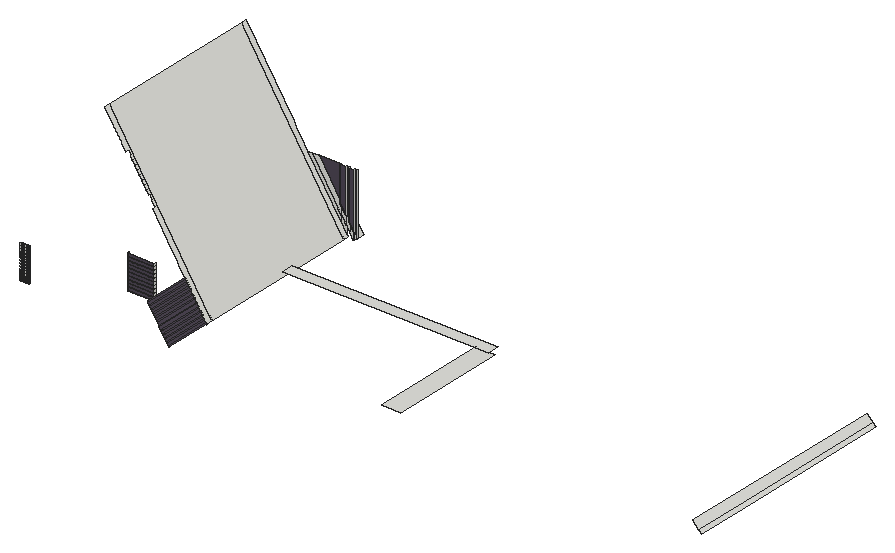
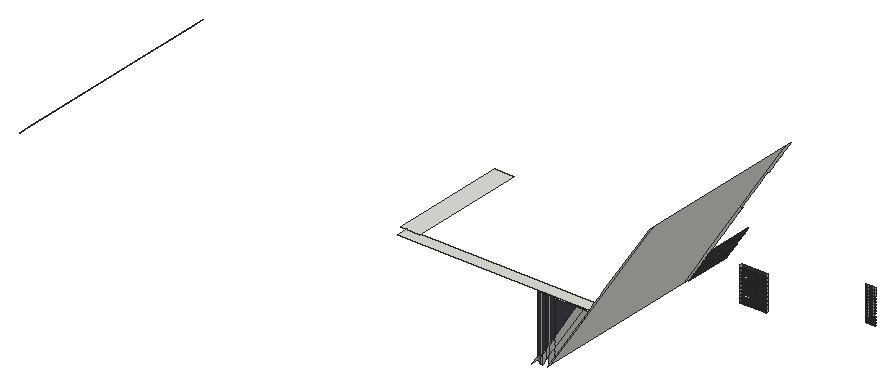
# SketchUp Ruby script. Lengths in inches.
U = 1.inch
M = Sketchup.active_model
def pt(a) = Geom::Point3d.new(a.map { |v| v * U })
def face(e, loops, mat)
  f = e.add_face(loops[0].map { |a| pt(a) })
  loops[1..].each { |l| e.add_face(l.map { |a| pt(a) }).erase! }
  f.material = f.back_material = mat if mat
  f
end
# faces: each face lists its corners as indices into pts; further lists are holes
def faces(e, pts, list, mat = nil) = list.each { |f| face(e, (f[0].is_a?(Array) ? f : [f]).map { |l| l.map { |i| pts[i] } }, mat) }
# xy, xz, yz: faces in a plane at the given z, y or x. An outline is a flat list of corners, or four numbers for a rectangle; further outlines are holes
def ring(l) = l.size == 4 ? [[l[0], l[1]], [l[2], l[1]], [l[2], l[3]], [l[0], l[3]]] : l.each_slice(2).to_a
def flat(e, list, mat, &to3) = list.each { |f| face(e, (f[0].is_a?(Array) ? f : [f]).map { |l| ring(l).map { |u, v| to3.(u, v) } }, mat) }
def xy(e, z, list, mat = nil) = flat(e, list, mat) { |x, y| [x, y, z] }
def xz(e, y, list, mat = nil) = flat(e, list, mat) { |x, z| [x, y, z] }
def yz(e, x, list, mat = nil) = flat(e, list, mat) { |y, z| [x, y, z] }
def lines(e, pts, list) = list.each { |a, b| e.add_line(pt(pts[a]), pt(pts[b])) }
# prism: a flat outline (further loops are holes) pulled along v
def prism(e, loops, v, mat = nil)
  f = face(e, loops, mat); d = Geom::Vector3d.new(v.map { |x| x * U })
  f.pushpull(f.normal.samedirection?(d) ? d.length : -d.length)
end
def box(e, o, s, mat = nil) = prism(e, [[o, [o[0] + s[0], o[1], o[2]], [o[0] + s[0], o[1] + s[1], o[2]], [o[0], o[1] + s[1], o[2]]]], [0, 0, s[2]], mat)
def at(x, y, z, deg = 0) = Geom::Transformation.translation(pt([x, y, z])) * Geom::Transformation.rotation(ORIGIN, Z_AXIS, deg.degrees)
def axes(o, x, y, z) = Geom::Transformation.new([*x, 0, *y, 0, *z, 0, *pt(o).to_a, 1])
def part(name) = M.definitions.add(name)
# library, detail: a bought-in or finely detailed component or shape, given as its bounding box
def library(name, o, s) = part(name).tap { |d| box(d.entities, o, s) }
def detail(e, o, s) = box(e.add_group.entities, o, s)
def put(e, d, t, mat = nil) = e.add_instance(d, t).tap { |i| i.material = mat if mat }
def group(e, t, mat = nil) = e.add_group.tap { |g| g.transformation = t; g.material = mat if mat }.entities
root = M.entities
M.materials.add("[Color M06]").color = [79, 71, 84]
xy(root,265.77,[[488.12,480.14,490.43,480.77],[491.03,480.14,493.35,480.77],[493.94,480.14,496.26,480.77],[496.86,480.14,499.17,480.77]])
xy(root,267.02,[[578.05,523.75,609.02,526.125]])
xy(root,267.83,[[578.05,523.75,609.02,526.125]])
xy(root,268.09,[[488.12,480.14,490.43,480.77],[491.03,480.14,493.35,480.77],[493.94,480.14,496.26,480.77],[496.86,480.14,499.17,480.77]])
xy(root,268.82,[[488.15,480.14,490.46,480.77],[491.0625,480.14,493.375,480.77],[493.97,480.14,496.29,480.77],[496.89,480.14,499.2,480.77]])
xy(root,270.95,[[578.05,523.75,609.02,526.125]])
xy(root,271.13,[[488.15,480.14,490.46,480.77],[491.0625,480.14,493.375,480.77],[493.97,480.14,496.29,480.77],[496.89,480.14,499.2,480.77]])
xy(root,271.76,[[578.05,523.75,609.02,526.125]])
xy(root,271.86,[[488.18,480.14,490.49,480.77],[491.09,480.14,493.4,480.77],[494,480.14,496.32,480.77],[496.91,480.14,499.23,480.77]])
xy(root,274.17,[[488.18,480.14,490.49,480.77],[491.09,480.14,493.4,480.77],[494,480.14,496.32,480.77],[496.91,480.14,499.23,480.77]])
xy(root,274.89,[[578.05,523.75,609.02,526.125]])
xy(root,274.91,[[488.21,480.14,490.52,480.77],[491.12,480.14,493.43,480.77],[494.03,480.14,496.34,480.77],[496.94,480.14,499.26,480.77]])
xy(root,275.7,[[578.05,523.75,609.02,526.125]])
xy(root,277.22,[[488.21,480.14,490.52,480.77],[491.12,480.14,493.43,480.77],[494.03,480.14,496.34,480.77],[496.94,480.14,499.26,480.77]])
xy(root,277.95,[[488.24,480.14,490.55,480.77],[491.15,480.14,493.46,480.77],[494.0625,480.14,496.375,480.77],[496.97,480.14,499.29,480.77]])
xy(root,278.1875,[[901.22,487.3125,923.77,623.84],[677.53,623.84,916.77,636.82]])
xy(root,278.83,[[578.05,523.75,609.02,526.125]])
xy(root,279.64,[[578.05,523.75,609.02,526.125]])
xy(root,280.26,[[488.24,480.14,490.55,480.77],[491.15,480.14,493.46,480.77],[494.0625,480.14,496.375,480.77],[496.97,480.14,499.29,480.77]])
xy(root,281,[[488.27,480.14,490.58,480.77],[491.18,480.14,493.49,480.77],[494.09,480.14,496.4,480.77],[497,480.14,499.3125,480.77]])
xy(root,282.77,[[578.05,523.75,609.02,526.125]])
xy(root,283.31,[[488.27,480.14,490.58,480.77],[491.18,480.14,493.49,480.77],[494.09,480.14,496.4,480.77],[497,480.14,499.3125,480.77]])
xy(root,283.58,[[578.05,523.75,609.02,526.125]],"[Color M06]")
xy(root,284.04,[[488.29,480.14,490.61,480.77],[491.21,480.14,493.52,480.77],[494.12,480.14,496.43,480.77],[497.03,480.14,499.34,480.77]])
xy(root,286.35,[[488.29,480.14,490.61,480.77],[491.21,480.14,493.52,480.77],[494.12,480.14,496.43,480.77],[497.03,480.14,499.34,480.77]])
xy(root,286.7,[[578.05,523.75,609.02,526.125]])
xy(root,287.09,[[488.32,480.14,490.64,480.77],[491.24,480.14,493.55,480.77],[494.15,480.14,496.46,480.77],[497.06,480.14,499.37,480.77]])
xy(root,287.51,[[578.05,523.75,609.02,526.125]],"[Color M06]")
xy(root,289.4,[[488.32,480.14,490.64,480.77],[491.24,480.14,493.55,480.77],[494.15,480.14,496.46,480.77],[497.06,480.14,499.37,480.77]])
xy(root,290.13,[[488.35,480.14,490.67,480.77],[491.26,480.14,493.58,480.77],[494.18,480.14,496.49,480.77],[497.09,480.14,499.4,480.77]])
xy(root,290.64,[[578.05,523.75,609.02,526.125]])
xy(root,291.45,[[578.05,523.75,609.02,526.125]],"[Color M06]")
xy(root,292.44,[[488.35,480.14,490.67,480.77],[491.26,480.14,493.58,480.77],[494.18,480.14,496.49,480.77],[497.09,480.14,499.4,480.77]])
xy(root,293.18,[[488.38,480.14,490.69,480.77],[491.29,480.14,493.61,480.77],[494.21,480.14,496.52,480.77],[497.12,480.14,499.43,480.77]])
xy(root,294.58,[[578.05,523.75,609.02,526.125]])
xy(root,295.39,[[578.05,523.75,609.02,526.125]])
xy(root,295.49,[[488.38,480.14,490.69,480.77],[491.29,480.14,493.61,480.77],[494.21,480.14,496.52,480.77],[497.12,480.14,499.43,480.77]])
xy(root,296.22,[[488.41,480.14,490.72,480.77],[491.32,480.14,493.64,480.77],[494.23,480.14,496.55,480.77],[497.15,480.14,499.46,480.77]])
xy(root,298.52,[[578.05,523.75,609.02,526.125]])
xy(root,298.53,[[488.41,480.14,490.72,480.77],[491.32,480.14,493.64,480.77],[494.23,480.14,496.55,480.77],[497.15,480.14,499.46,480.77]])
xy(root,299.27,[[488.44,480.14,490.75,480.77],[491.35,480.14,493.66,480.77],[494.26,480.14,496.58,480.77],[497.18,480.14,499.49,480.77]])
xy(root,299.33,[[578.05,523.75,609.02,526.125]])
xy(root,301.58,[[488.44,480.14,490.75,480.77],[491.35,480.14,493.66,480.77],[494.26,480.14,496.58,480.77],[497.18,480.14,499.49,480.77]])
xy(root,302.31,[[488.47,480.14,490.78,480.77],[491.38,480.14,493.69,480.77],[494.29,480.14,496.61,480.77],[497.2,480.14,499.52,480.77]])
xy(root,302.45,[[578.05,523.75,609.02,526.125]])
xy(root,303.26,[[578.05,523.75,609.02,526.125]])
xy(root,304.62,[[488.47,480.14,490.78,480.77],[491.38,480.14,493.69,480.77],[494.29,480.14,496.61,480.77],[497.2,480.14,499.52,480.77]])
xz(root,521.5625,[[671.46,265.95,671.2,266.36,671.46,266.53],[670.66,267.19,670.93,267.36,669.23,270,668.97,269.84],[668.4375,270.67,668.7,270.83,667.01,273.48,666.74,273.31],[666.21,274.14,666.47,274.31,664.78,276.95,664.52,276.78],[663.98,277.61,664.25,277.78,662.55,280.42,662.29,280.25],
  [661.76,281.08,662.02,281.25,660.33,283.89,660.0625,283.73],[659.53,284.56,659.8,284.72,658.1,287.37,657.84,287.2],[657.31,288.03,657.57,288.2,655.875,290.84,655.61,290.67],[655.08,291.5,653.39,294.14,653.65,294.3125,655.34,291.67],[652.85,294.97,653.12,295.14,651.42,297.79,651.16,297.62],
  [650.625,298.45,650.89,298.61,649.2,301.26,648.93,301.09],[648.3,301.85,648.66,302.09,646.97,304.73,646.6,304.49]])
xz(root,523.75,[[578.05,267.83,609.02,270.95],[578.05,271.76,609.02,274.89],[578.05,275.7,609.02,278.83],[578.05,279.64,609.02,282.77],[578.05,283.58,609.02,286.7],
  [578.05,287.51,609.02,290.64],[578.05,291.45,609.02,294.58],[578.05,295.39,609.02,298.52],[578.05,299.33,609.02,302.45],[578.05,303.26,609.02,306.39]],"[Color M06]")
xz(root,526.125,[[578.05,302.45,609.02,303.26]])
xz(root,526.125,[[578.05,267.02,609.02,267.83],[578.05,270.95,609.02,271.76],[578.05,274.89,609.02,275.7],[578.05,278.83,609.02,279.64],[578.05,282.77,609.02,283.58],
  [578.05,286.7,609.02,287.51],[578.05,290.64,609.02,291.45],[578.05,294.58,609.02,295.39],[578.05,298.52,609.02,299.33]],"[Color M06]")
xz(root,724.8125,[[679.27,274.85,679.27,340.125,673.19,340.125,673.19,284.33,677.53,277.56],[669.77,289.67,669.77,340.125,663.69,340.125,663.69,299.15]],"[Color M06]")
xz(root,726.125,[[677.53,265.98,677.53,277.56,673.19,284.33,673.19,272.75],[677.53,265.98,679.27,267.09,679.27,274.85,677.53,277.56],[679.27,267.09,679.27,274.85,682.69,269.51,682.69,269.29],[669.77,269.17,669.77,278.09,663.69,287.57,663.69,278.65],[682.69,269.29,682.79,269.35,682.69,269.51],
  [673.19,272.75,673.19,284.33,669.77,289.67,669.77,278.09],[669.77,278.09,669.77,289.67,663.69,299.15,663.69,287.57],[663.69,278.65,663.69,287.57,629.99,340.125,624.28,340.125],[663.69,287.57,663.69,299.15,637.42,340.125,629.99,340.125]])
xz(root,726.125,[[682.69,269.51,682.69,340.125,679.27,340.125,679.27,274.85],[673.19,284.33,673.19,340.125,669.77,340.125,669.77,289.67],[663.69,299.15,663.69,340.125,637.42,340.125]],"[Color M06]")
yz(root,488.41,[[480.14,296.22,480.77,298.53]])
yz(root,488.44,[[480.14,299.27,480.77,301.58]])
yz(root,488.47,[[480.14,302.31,480.77,304.62]])
yz(root,490.43,[[480.14,265.77,480.77,268.09]])
yz(root,490.46,[[480.14,268.82,480.77,271.13]])
yz(root,490.49,[[480.14,271.86,480.77,274.17]])
yz(root,490.52,[[480.14,274.91,480.77,277.22]])
yz(root,490.55,[[480.14,277.95,480.77,280.26]])
yz(root,490.58,[[480.14,281,480.77,283.31]])
yz(root,490.61,[[480.14,284.04,480.77,286.35]])
yz(root,490.64,[[480.14,287.09,480.77,289.4]])
yz(root,490.67,[[480.14,290.13,480.77,292.44]])
yz(root,490.69,[[480.14,293.18,480.77,295.49]])
yz(root,490.72,[[480.14,296.22,480.77,298.53]])
yz(root,490.75,[[480.14,299.27,480.77,301.58]])
yz(root,490.78,[[480.14,302.31,480.77,304.62]])
yz(root,491.03,[[480.14,265.77,480.77,268.09]])
yz(root,491.0625,[[480.14,268.82,480.77,271.13]])
yz(root,491.09,[[480.14,271.86,480.77,274.17]])
yz(root,491.12,[[480.14,274.91,480.77,277.22]])
yz(root,491.15,[[480.14,277.95,480.77,280.26]])
yz(root,491.18,[[480.14,281,480.77,283.31]])
yz(root,491.21,[[480.14,284.04,480.77,286.35]])
yz(root,491.24,[[480.14,287.09,480.77,289.4]])
yz(root,491.26,[[480.14,290.13,480.77,292.44]])
yz(root,491.29,[[480.14,293.18,480.77,295.49]])
yz(root,491.32,[[480.14,296.22,480.77,298.53]])
yz(root,491.35,[[480.14,299.27,480.77,301.58]])
yz(root,491.38,[[480.14,302.31,480.77,304.62]])
yz(root,493.35,[[480.14,265.77,480.77,268.09]])
yz(root,493.375,[[480.14,268.82,480.77,271.13]])
yz(root,493.4,[[480.14,271.86,480.77,274.17]])
yz(root,493.43,[[480.14,274.91,480.77,277.22]])
yz(root,493.46,[[480.14,277.95,480.77,280.26]])
yz(root,493.49,[[480.14,281,480.77,283.31]])
yz(root,493.52,[[480.14,284.04,480.77,286.35]])
yz(root,493.55,[[480.14,287.09,480.77,289.4]])
yz(root,493.58,[[480.14,290.13,480.77,292.44]])
yz(root,493.61,[[480.14,293.18,480.77,295.49]])
yz(root,493.64,[[480.14,296.22,480.77,298.53]])
yz(root,493.66,[[480.14,299.27,480.77,301.58]])
yz(root,493.69,[[480.14,302.31,480.77,304.62]])
yz(root,493.94,[[480.14,265.77,480.77,268.09]])
yz(root,493.97,[[480.14,268.82,480.77,271.13]])
yz(root,494,[[480.14,271.86,480.77,274.17]])
yz(root,494.03,[[480.14,274.91,480.77,277.22]])
yz(root,494.0625,[[480.14,277.95,480.77,280.26]])
yz(root,494.09,[[480.14,281,480.77,283.31]])
yz(root,494.12,[[480.14,284.04,480.77,286.35]])
yz(root,494.15,[[480.14,287.09,480.77,289.4]])
yz(root,494.18,[[480.14,290.13,480.77,292.44]])
yz(root,494.21,[[480.14,293.18,480.77,295.49]])
yz(root,494.23,[[480.14,296.22,480.77,298.53]])
yz(root,494.26,[[480.14,299.27,480.77,301.58]])
yz(root,494.29,[[480.14,302.31,480.77,304.62]])
yz(root,496.26,[[480.14,265.77,480.77,268.09]])
yz(root,496.29,[[480.14,268.82,480.77,271.13]])
yz(root,496.32,[[480.14,271.86,480.77,274.17]])
yz(root,496.34,[[480.14,274.91,480.77,277.22]])
yz(root,496.375,[[480.14,277.95,480.77,280.26]])
yz(root,496.4,[[480.14,281,480.77,283.31]])
yz(root,496.43,[[480.14,284.04,480.77,286.35]])
yz(root,496.46,[[480.14,287.09,480.77,289.4]])
yz(root,496.49,[[480.14,290.13,480.77,292.44]])
yz(root,496.52,[[480.14,293.18,480.77,295.49]])
yz(root,496.55,[[480.14,296.22,480.77,298.53]])
yz(root,496.58,[[480.14,299.27,480.77,301.58]])
yz(root,496.61,[[480.14,302.31,480.77,304.62]])
yz(root,496.86,[[480.14,265.77,480.77,268.09]])
yz(root,496.89,[[480.14,268.82,480.77,271.13]])
yz(root,496.91,[[480.14,271.86,480.77,274.17]])
yz(root,496.94,[[480.14,274.91,480.77,277.22]])
yz(root,496.97,[[480.14,277.95,480.77,280.26]])
yz(root,497,[[480.14,281,480.77,283.31]])
yz(root,497.03,[[480.14,284.04,480.77,286.35]])
yz(root,497.06,[[480.14,287.09,480.77,289.4]])
yz(root,497.09,[[480.14,290.13,480.77,292.44]])
yz(root,497.12,[[480.14,293.18,480.77,295.49]])
yz(root,497.15,[[480.14,296.22,480.77,298.53]])
yz(root,497.18,[[480.14,299.27,480.77,301.58]])
yz(root,497.2,[[480.14,302.31,480.77,304.62]])
yz(root,499.17,[[480.14,265.77,480.77,268.09]])
yz(root,499.2,[[480.14,268.82,480.77,271.13]])
yz(root,499.23,[[480.14,271.86,480.77,274.17]])
yz(root,499.26,[[480.14,274.91,480.77,277.22]])
yz(root,499.29,[[480.14,277.95,480.77,280.26]])
yz(root,499.3125,[[480.14,281,480.77,283.31]])
yz(root,499.34,[[480.14,284.04,480.77,286.35]])
yz(root,499.37,[[480.14,287.09,480.77,289.4]])
yz(root,499.4,[[480.14,290.13,480.77,292.44]])
yz(root,499.43,[[480.14,293.18,480.77,295.49]])
yz(root,499.46,[[480.14,296.22,480.77,298.53]])
yz(root,499.49,[[480.14,299.27,480.77,301.58]])
yz(root,499.52,[[480.14,302.31,480.77,304.62]])
yz(root,578.05,[[523.75,267.83,526.125,270.95],[523.75,271.76,526.125,274.89],[523.75,275.7,526.125,278.83],[523.75,279.64,526.125,282.77],[523.75,283.58,526.125,286.7],
  [523.75,287.51,526.125,290.64],[523.75,291.45,526.125,294.58],[523.75,295.39,526.125,298.52],[523.75,299.33,526.125,302.45],[523.75,303.26,526.125,306.39]])
yz(root,609.02,[[523.75,267.83,526.125,270.95],[523.75,271.76,526.125,274.89],[523.75,275.7,526.125,278.83],[523.75,279.64,526.125,282.77],[523.75,283.58,526.125,286.7],
  [523.75,287.51,526.125,290.64],[523.75,291.45,526.125,294.58],[523.75,295.39,526.125,298.52],[523.75,299.33,526.125,302.45],[523.75,303.26,526.125,306.39]])
yz(root,663.69,[[724.8125,299.15,726.125,340.125]])
yz(root,669.77,[[724.8125,289.67,726.125,340.125]])
yz(root,673.19,[[724.8125,284.33,726.125,340.125]])
yz(root,679.27,[[724.8125,274.85,726.125,340.125]])
yz(root,682.69,[[724.8125,269.51,726.125,340.125]])
p = [[671.46,467.1875,266.53],[671.46,521.5625,266.53],[671.2,521.5625,266.36],[671.2,467.1875,266.36],[670.93,467.1875,267.36],[670.93,521.5625,267.36],
  [671.46,528.48,266.53],[553.56,528.48,450.4375],[553.56,521.5625,450.4375],[553.9375,521.5625,449.84],[555.125,521.5625,447.99],[555.68,521.5625,447.125],
  [556.13,521.5625,446.42],[557.32,521.5625,444.57],[557.87,521.5625,443.7],[558.32,521.5625,443],[559.51,521.5625,441.15],[560.0625,521.5625,440.28],
  [560.51,521.5625,439.58],[561.7,521.5625,437.73],[562.26,521.5625,436.86],[562.71,521.5625,436.16],[563.89,521.5625,434.31],[564.45,521.5625,433.44],
  [564.9,521.5625,432.74],[566.09,521.5625,430.89],[566.64,521.5625,430.02],[567.09,521.5625,429.32],[568.28,521.5625,427.47],[568.83,521.5625,426.6],
  [569.28,521.5625,425.9],[570.47,521.5625,424.05],[571.03,521.5625,423.18],[571.48,521.5625,422.48],[572.66,521.5625,420.63],[573.22,521.5625,419.76],
  [573.67,521.5625,419.0625],[574.86,521.5625,417.21],[575.41,521.5625,416.34],[575.86,521.5625,415.64],[577.05,521.5625,413.79],[577.61,521.5625,412.92],
  [578.05,521.5625,412.22],[578.05,526.125,412.22],[578.12,526.125,412.12],[580.125,526.125,409],[581,526.125,407.62],[581,524.25,407.62],
  [583.01,524.25,404.5],[583.01,526.125,404.5],[583.73,526.125,403.37],[583.73,524.25,403.37],[585.73,524.25,400.25],[585.73,526.125,400.25],
  [586.45,526.125,399.12],[586.45,524.25,399.12],[588.46,524.25,396],[588.46,526.125,396],[589.18,526.125,394.87],[589.18,524.25,394.87],
  [591.18,524.25,391.75],[591.18,526.125,391.75],[591.9,526.125,390.62],[591.9,524.25,390.62],[593.91,524.25,387.5],[593.91,526.125,387.5],
  [594.63,526.125,386.37],[594.63,524.25,386.37],[596.63,524.25,383.25],[596.63,526.125,383.25],[597.35,526.125,382.12],[597.35,524.25,382.12],
  [599.36,524.25,379],[599.36,526.125,379],[600.08,526.125,377.87],[600.08,524.25,377.87],[602.08,524.25,374.75],[602.08,526.125,374.75],
  [602.8,526.125,373.62],[604.81,526.125,370.5],[605.53,526.125,369.37],[605.53,524.25,369.37],[607.53,524.25,366.25],[607.53,526.125,366.25],
  [608.25,526.125,365.12],[609.02,526.125,363.92],[609.02,524.25,363.92],[609.02,521.5625,363.92],[610.21,521.5625,362.07],[610.84,521.5625,361.08],
  [610.9,521.5625,360.99],[612.54,521.5625,358.4375],[613.17,521.5625,357.45],[614.86,521.5625,354.81],[615.5,521.5625,353.82],[617.19,521.5625,351.18],
  [617.82,521.5625,350.19],[619.52,521.5625,347.55],[620.15,521.5625,346.56],[621.85,521.5625,343.92],[622.48,521.5625,342.93],[624.17,521.5625,340.29],
  [624.28,521.5625,340.125],[624.71,521.5625,339.46],[626.4,521.5625,336.8125],[626.93,521.5625,335.98],[628.625,521.5625,333.34],[629.16,521.5625,332.51],
  [630.85,521.5625,329.87],[631.39,521.5625,329.04],[633.08,521.5625,326.4],[633.61,521.5625,325.57],[635.31,521.5625,322.92],[635.84,521.5625,322.09],
  [637.53,521.5625,319.45],[638.0625,521.5625,318.62],[639.76,521.5625,315.98],[640.29,521.5625,315.15],[641.98,521.5625,312.51],[642.52,521.5625,311.68],
  [644.21,521.5625,309.03],[644.74,521.5625,308.2],[646.4375,521.5625,305.56],[646.97,521.5625,304.73],[648.66,521.5625,302.09],[649.2,521.5625,301.26],
  [650.89,521.5625,298.61],[651.42,521.5625,297.79],[653.12,521.5625,295.14],[653.65,521.5625,294.3125],[655.34,521.5625,291.67],[655.875,521.5625,290.84],
  [657.57,521.5625,288.2],[658.1,521.5625,287.37],[659.8,521.5625,284.72],[660.33,521.5625,283.89],[662.02,521.5625,281.25],[662.55,521.5625,280.42],
  [664.25,521.5625,277.78],[664.78,521.5625,276.95],[666.47,521.5625,274.31],[667.01,521.5625,273.48],[668.7,521.5625,270.83],[669.23,521.5625,270],
  [671.46,719.59,266.53],[553.56,719.59,450.4375],[624.28,726.125,340.125],[663.69,726.125,278.65],[669.77,726.125,269.17],[671.46,726.125,266.53],
  [553.56,726.125,450.4375],[608.37,726.125,364.9375],[611.36,726.125,360.28],[617.83,726.125,350.1875],[668.97,521.5625,269.84],[670.66,521.5625,267.19],
  [670.66,467.1875,267.19],[668.97,467.1875,269.84],[682.79,726.125,269.35],[682.69,726.125,269.51],[682.69,724.8125,269.51],[682.79,724.8125,269.35],
  [679.27,726.125,274.85],[677.53,726.125,277.56],[677.53,734.4375,277.56],[682.79,734.4375,269.35],[669.23,467.1875,270],[668.7,467.1875,270.83],
  [666.74,521.5625,273.31],[668.4375,521.5625,270.67],[668.4375,467.1875,270.67],[666.74,467.1875,273.31],[667.01,467.1875,273.48],[666.47,467.1875,274.31],
  [664.52,521.5625,276.78],[666.21,521.5625,274.14],[666.21,467.1875,274.14],[664.52,467.1875,276.78],[677.53,724.8125,277.56],[679.27,724.8125,274.85],
  [664.78,467.1875,276.95],[664.25,467.1875,277.78],[662.29,521.5625,280.25],[663.98,521.5625,277.61],[663.98,467.1875,277.61],[662.29,467.1875,280.25],
  [673.19,726.125,284.33],[673.19,724.8125,284.33],[662.55,467.1875,280.42],[662.02,467.1875,281.25],[660.0625,521.5625,283.73],[661.76,521.5625,281.08],
  [661.76,467.1875,281.08],[660.0625,467.1875,283.73],[660.33,467.1875,283.89],[659.8,467.1875,284.72],[657.84,521.5625,287.2],[659.53,521.5625,284.56],
  [659.53,467.1875,284.56],[657.84,467.1875,287.2],[658.1,467.1875,287.37],[657.57,467.1875,288.2],[655.61,521.5625,290.67],[657.31,521.5625,288.03],
  [657.31,467.1875,288.03],[655.61,467.1875,290.67],[1288.59,467.1875,289.56],[1285.45,467.1875,292.52],[1285.45,528.48,292.52],[1285.45,719.2,292.52],
  [1288.59,719.2,289.56],[1288.59,521.5625,289.56],[669.77,726.125,289.67],[663.69,726.125,299.15],[663.69,724.8125,299.15],[669.77,724.8125,289.67],
  [655.875,467.1875,290.84],[655.34,467.1875,291.67],[653.39,521.5625,294.14],[655.08,521.5625,291.5],[655.08,467.1875,291.5],[653.39,467.1875,294.14],
  [1277.91,467.1875,299.61],[1277.91,719.2,299.61],[653.65,467.1875,294.3125],[653.12,467.1875,295.14],[651.16,521.5625,297.62],[652.85,521.5625,294.97],
  [652.85,467.1875,294.97],[651.16,467.1875,297.62],[651.42,467.1875,297.79],[650.89,467.1875,298.61],[648.93,521.5625,301.09],[650.625,521.5625,298.45],
  [650.625,467.1875,298.45],[648.93,467.1875,301.09],[649.2,467.1875,301.26],[648.66,467.1875,302.09],[646.6,521.5625,304.49],[648.3,521.5625,301.85],
  [648.3,467.1875,301.85],[646.6,467.1875,304.49],[646.97,467.1875,304.73],[646.4375,467.1875,305.56]]
faces(root,p,[[0,1,2,3],[6,7,8,9,10,11,12,13,14,15,16,17,18,19,20,21,22,23,24,25,26,27,28,29,30,31,32,33,34,35,36,37,38,39,40,41,42,43,44,45,46,47,48,49,50,51,52,53,54,55,56,57,58,59,60,61,62,63,64,65,66,67,68,69,70,71,72,73,74,75,76,77,78,79,80,81,82,83,84,85,86,87,88,89,90,91,92,93,94,95,96,97,98,99,100,101,102,103,104,105,106,107,108,109,110,111,112,113,114,115,116,117,118,119,120,121,122,123,124,125,126,127,128,129,130,131,132,133,134,135,136,137,138,139,140,141,142,143,5,1],[144,6,7,145],[146,147,148,149,144,145,150,151,152,153],[5,4,156,155],[158,159,160,161],[162,163,164,165,158,159],[166,143,154,157],
  [142,167,170,169],[172,141,168,171],[140,173,176,175],[162,163,178,179],[180,139,174,177],[138,181,184,183],[163,186,187,178],[188,137,182,185],
  [136,189,192,191],[194,135,190,193],[134,195,198,197],[200,133,196,199],[132,201,204,203],[206,207,208,209,210,211],[212,213,214,215],[216,131,202,205],
  [130,217,220,219],[207,222,223,209,208],[224,129,218,221],[128,225,228,227],[230,127,226,229],[126,231,234,233],[236,125,232,235],[124,237,240,239],
  [242,123,238,241]])
faces(root,p,[[0,4,5,1],[154,155,156,157],[166,167,142,143],[168,169,170,171],[172,173,140,141],[174,175,176,177],[180,181,138,139],[182,183,184,185],
  [188,189,136,137],[190,191,192,193],[194,195,134,135],[196,197,198,199],[200,201,132,133],[202,203,204,205],[216,217,130,131],[218,219,220,221],
  [224,225,128,129],[226,227,228,229],[230,231,126,127],[232,233,234,235],[236,237,124,125],[238,239,240,241],[242,243,122,123]],"[Color M06]")
